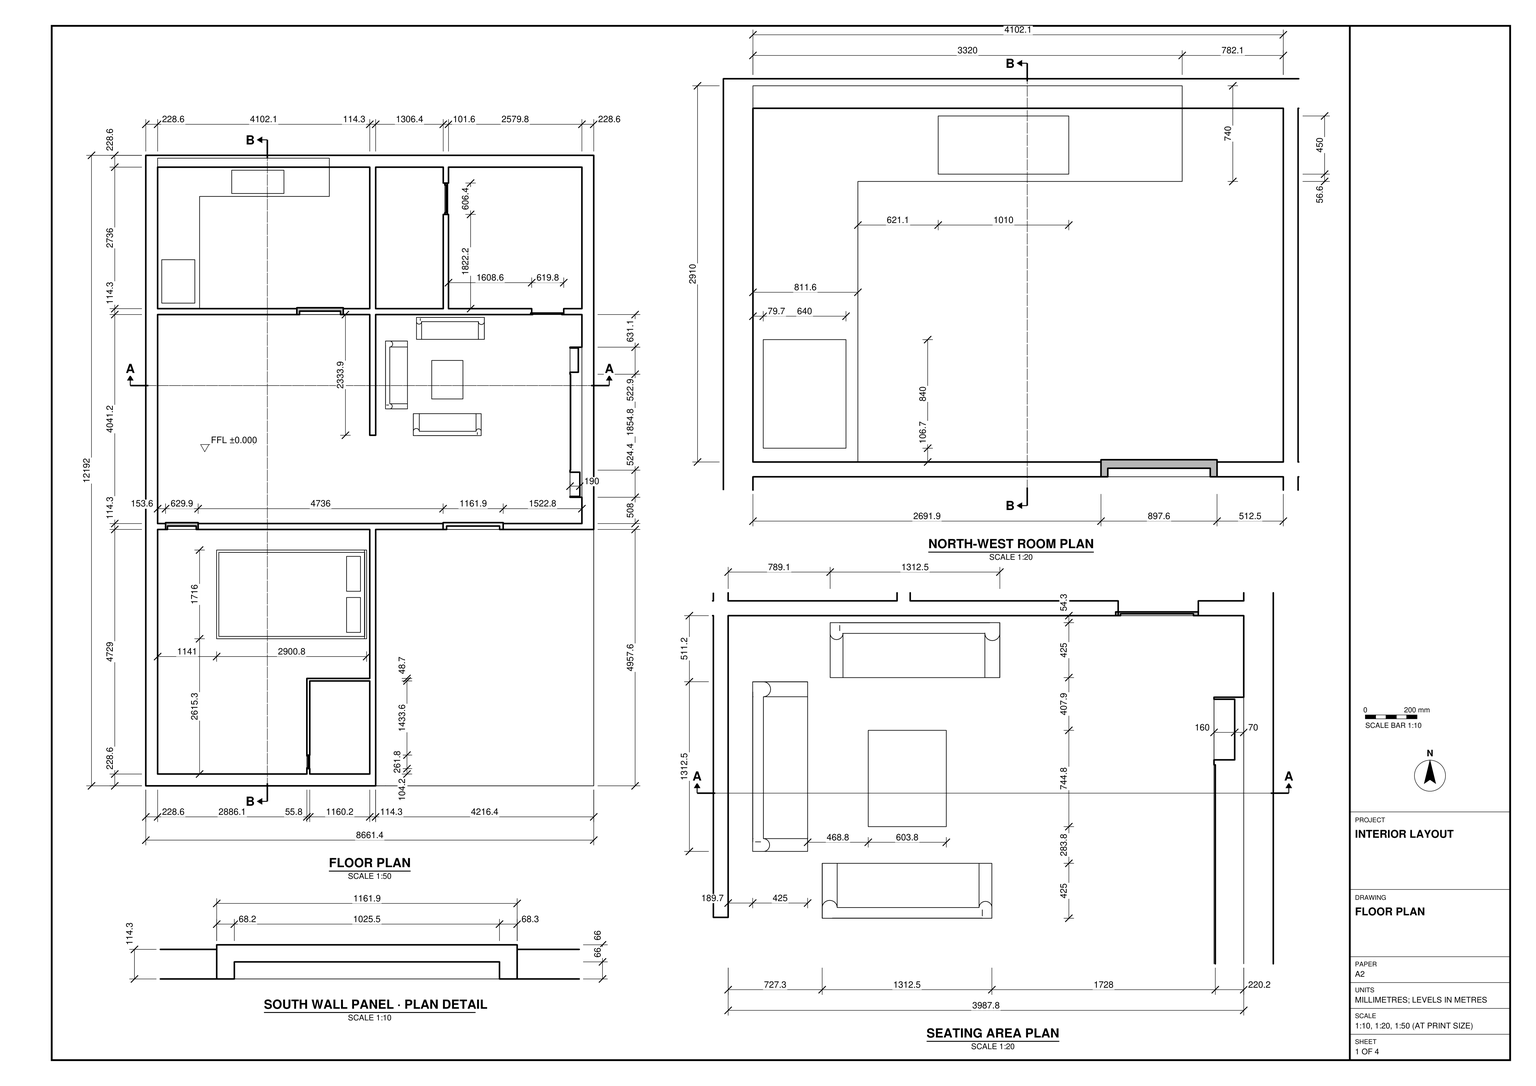
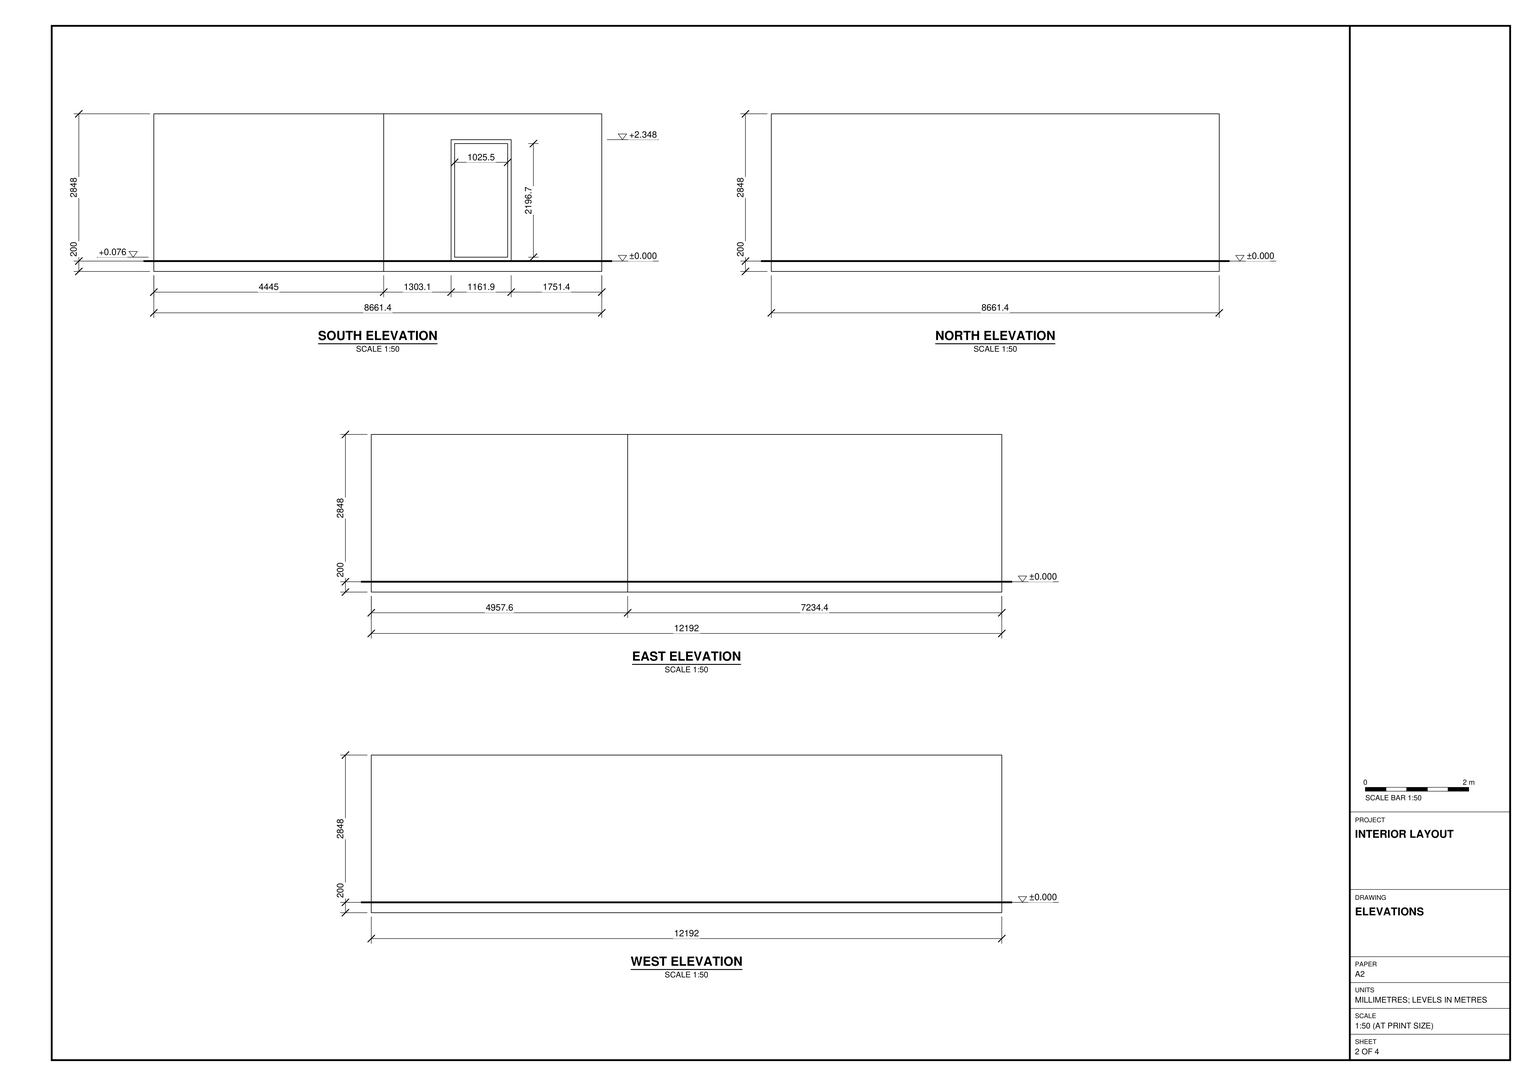
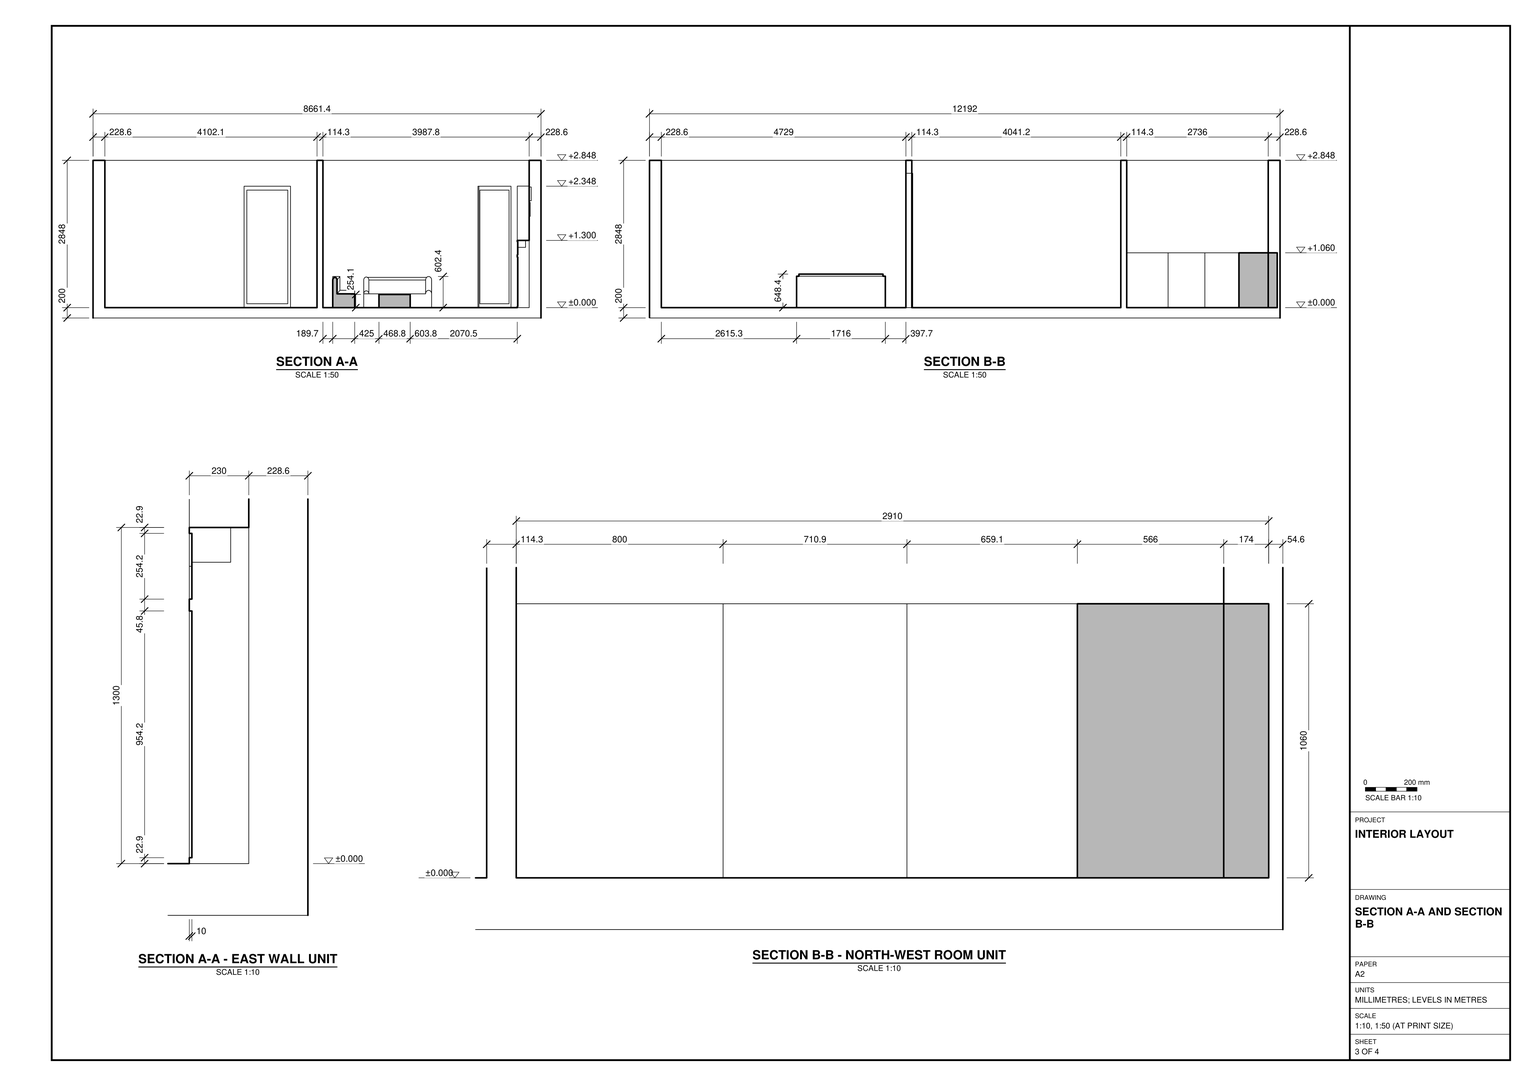
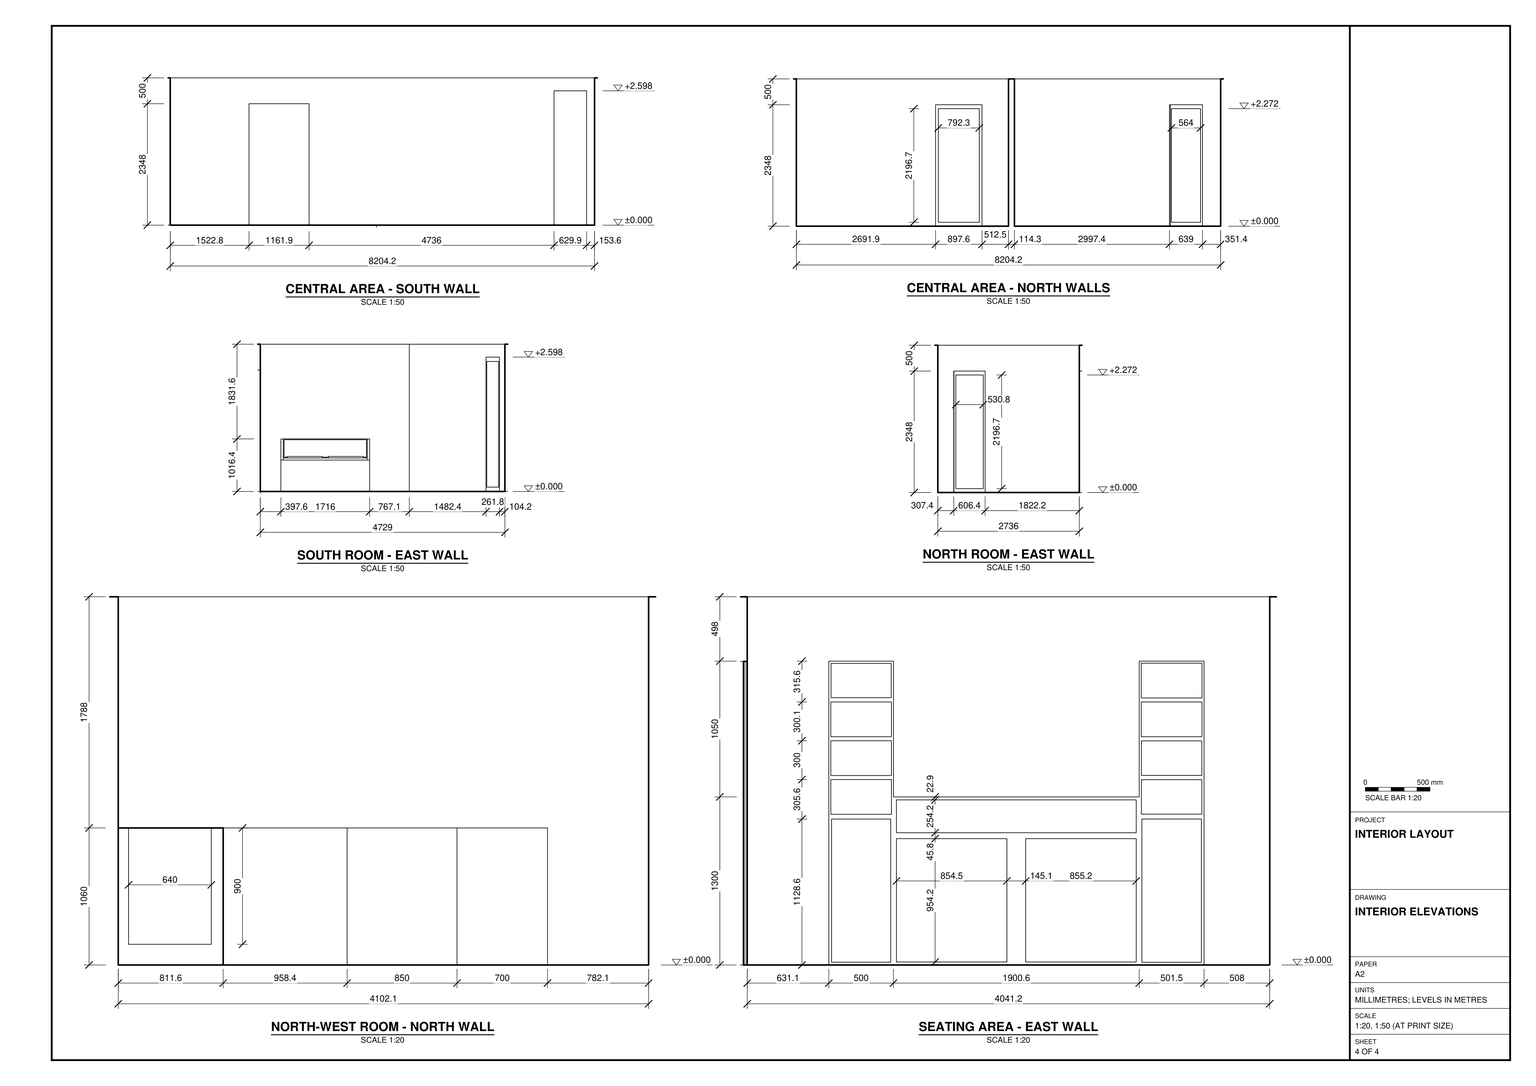
Build the interior in SketchUp from task_files/diagram_01.pdf. Work in millimetres. Set the finished floor at 0 mm and make the overall model 8661.4 mm east–west, 12192 mm north–south and 3048 mm high, including the 200 mm floor slab.

Follow the floor plan for the wall runs, thicknesses and openings. The northern row has a fitted room at the west end and two rooms to its east. In the central area, stop the dividing wall short of the south wall so the seating area remains connected to the space on its west side. Carry the bedroom south on the west side of the plan, with the bed oriented east–west and the short return partition in the bedroom corner.

Use the enlarged plans and sections to build the L-shaped unit in the north-west room, the shallow unit on the east wall and the framed panel in the south wall. Arrange the three sofas around the rectangular table as drawn. Decor and loose items shown may be any suitable library components. Keep the slab and walls separate from one another and from the fit-out. Make each furniture or joinery piece a group or component and use components for repeated parts. Save one SketchUp model as output_files/furnished_single_storey_interior_with_joinery.skp.

# SketchUp Ruby script. Lengths in millimetres.
U = 1.mm
M = Sketchup.active_model
def pt(a) = Geom::Point3d.new(a.map { |v| v * U })
def face(e, loops, mat)
  f = e.add_face(loops[0].map { |a| pt(a) })
  loops[1..].each { |l| e.add_face(l.map { |a| pt(a) }).erase! }
  f.material = f.back_material = mat if mat
  f
end
# faces: each face lists its corners as indices into pts; further lists are holes
def faces(e, pts, list, mat = nil) = list.each { |f| face(e, (f[0].is_a?(Array) ? f : [f]).map { |l| l.map { |i| pts[i] } }, mat) }
# xy, xz, yz: faces in a plane at the given z, y or x. An outline is a flat list of corners, or four numbers for a rectangle; further outlines are holes
def ring(l) = l.size == 4 ? [[l[0], l[1]], [l[2], l[1]], [l[2], l[3]], [l[0], l[3]]] : l.each_slice(2).to_a
def flat(e, list, mat, &to3) = list.each { |f| face(e, (f[0].is_a?(Array) ? f : [f]).map { |l| ring(l).map { |u, v| to3.(u, v) } }, mat) }
def xy(e, z, list, mat = nil) = flat(e, list, mat) { |x, y| [x, y, z] }
def xz(e, y, list, mat = nil) = flat(e, list, mat) { |x, z| [x, y, z] }
def yz(e, x, list, mat = nil) = flat(e, list, mat) { |y, z| [x, y, z] }
def lines(e, pts, list) = list.each { |a, b| e.add_line(pt(pts[a]), pt(pts[b])) }
# prism: a flat outline (further loops are holes) pulled along v
def prism(e, loops, v, mat = nil)
  f = face(e, loops, mat); d = Geom::Vector3d.new(v.map { |x| x * U })
  f.pushpull(f.normal.samedirection?(d) ? d.length : -d.length)
end
def box(e, o, s, mat = nil) = prism(e, [[o, [o[0] + s[0], o[1], o[2]], [o[0] + s[0], o[1] + s[1], o[2]], [o[0], o[1] + s[1], o[2]]]], [0, 0, s[2]], mat)
def at(x, y, z, deg = 0) = Geom::Transformation.translation(pt([x, y, z])) * Geom::Transformation.rotation(ORIGIN, Z_AXIS, deg.degrees)
def axes(o, x, y, z) = Geom::Transformation.new([*x, 0, *y, 0, *z, 0, *pt(o).to_a, 1])
def part(name) = M.definitions.add(name)
# library, detail: a bought-in or finely detailed component or shape, given as its bounding box
def library(name, o, s) = part(name).tap { |d| box(d.entities, o, s) }
def detail(e, o, s) = box(e.add_group.entities, o, s)
def put(e, d, t, mat = nil) = e.add_instance(d, t).tap { |i| i.material = mat if mat }
def group(e, t, mat = nil) = e.add_group.tap { |g| g.transformation = t; g.material = mat if mat }.entities
root = M.entities
M.materials.add("[Carpet Diamond Yellow]").color = [226, 217, 124]
M.materials.add("[Carpet Plush Charcoal]").color = [87, 87, 87]
M.materials.add("[Chipboard]").color = [205, 176, 119]
M.materials.add("[Color M06]").color = [86, 86, 86]
M.materials.add("[Marble Carrara Gold Floor Tile]").color = [225, 223, 217]
M.materials.add("[Plastic Red]").color = [245, 126, 1]
M.materials.add("[Resin Blue]").color = [171, 210, 241]
M.materials.add("[Resin Turquoise]").color = [117, 218, 223]
M.materials.add("[Wax 01]").color = [250, 213, 163]
M.materials.add("[Wax 02]").color = [173, 204, 163]
M.materials.add("[Wood Bamboo]").color = [177, 105, 43]
M.materials.add("[Wood Cherry Original]").color = [152, 86, 42]
c1 = part("Door panel")
xy(c1.entities,0,[[0,0,1570,60]],"[Wood Cherry Original]")
xy(c1.entities,92.1,[[92.1,0,1477.9,30]],"[Wood Cherry Original]")
xy(c1.entities,2767.9,[[92.1,0,1477.9,30]],"[Wood Cherry Original]")
xy(c1.entities,2860,[[0,0,1570,60]],"[Wood Cherry Original]")
xz(c1.entities,0,[[[0,0,1570,2860],[92.1,92.1,1477.9,2767.9]]],"[Wood Cherry Original]")
xz(c1.entities,30,[[92.1,92.1,1477.9,2767.9]],"[Wood Cherry Original]")
xz(c1.entities,60,[[0,0,1570,2860]],"[Wood Cherry Original]")
yz(c1.entities,0,[[0,0,60,2860]],"[Wood Cherry Original]")
yz(c1.entities,92.1,[[0,92.1,30,2767.9]],"[Wood Cherry Original]")
yz(c1.entities,1477.9,[[0,92.1,30,2767.9]],"[Wood Cherry Original]")
yz(c1.entities,1570,[[0,0,60,2860]],"[Wood Cherry Original]")
c2 = part("Bed with headboard")
xy(c2.entities,0,[[0,0,2860,5180]])
xy(c2.entities,1040,[[0,0,2860,0,2860,5104.1,2784.1,5104.1,2784.1,75.9,75.9,75.9,75.9,5104.1,0,5104.1]],"[Wood Cherry Original]")
xy(c2.entities,1110,[[[75.9,75.9,2784.1,5114.1],[205.2,4486.4,1330.2,4966.4],[1530.2,4486.4,2655.2,4966.4]]],"[Color M06]")
xy(c2.entities,1136.9,[[102.8,5104.1,2757.2,5114.1]])
xy(c2.entities,1160,[[205.2,4486.4,1330.2,4966.4],[1530.2,4486.4,2655.2,4966.4]],"[Color M06]")
xy(c2.entities,1713.1,[[102.8,5104.1,2757.2,5114.1]],"[Color M06]")
xy(c2.entities,1740,[[0,5104.1,75.9,5104.1,75.9,5114.1,2784.1,5114.1,2784.1,5104.1,2860,5104.1,2860,5180,0,5180]],"[Wood Cherry Original]")
xz(c2.entities,0,[[0,0,2860,1040]],"[Wood Cherry Original]")
xz(c2.entities,75.9,[[75.9,1040,2784.1,1110]],"[Color M06]")
xz(c2.entities,4486.4,[[205.2,1110,1330.2,1160],[1530.2,1110,2655.2,1160]],"[Color M06]")
xz(c2.entities,4966.4,[[205.2,1110,1330.2,1160],[1530.2,1110,2655.2,1160]])
xz(c2.entities,5104.1,[[102.8,1136.9,2757.2,1713.1]],"[Color M06]")
xz(c2.entities,5104.1,[[0,1040,75.9,1740],[2784.1,1040,2860,1740]],"[Wood Cherry Original]")
xz(c2.entities,5114.1,[[[75.9,1110,2784.1,1740],[102.8,1136.9,2757.2,1713.1]]],"[Wood Cherry Original]")
xz(c2.entities,5180,[[0,0,2860,1740]],"[Wood Cherry Original]")
yz(c2.entities,0,[[0,0,0,1040,5104.1,1040,5104.1,1740,5180,1740,5180,0]],"[Wood Cherry Original]")
yz(c2.entities,75.9,[[5104.1,1110,5114.1,1740]])
yz(c2.entities,75.9,[[75.9,1040,5104.1,1110]],"[Color M06]")
yz(c2.entities,102.8,[[5104.1,1136.9,5114.1,1713.1]],"[Color M06]")
yz(c2.entities,205.2,[[4486.4,1110,4966.4,1160]],"[Color M06]")
yz(c2.entities,1330.2,[[4486.4,1110,4966.4,1160]],"[Color M06]")
yz(c2.entities,1530.2,[[4486.4,1110,4966.4,1160]],"[Color M06]")
yz(c2.entities,2655.2,[[4486.4,1110,4966.4,1160]],"[Color M06]")
yz(c2.entities,2757.2,[[5104.1,1136.9,5114.1,1713.1]],"[Color M06]")
yz(c2.entities,2784.1,[[75.9,1040,5104.1,1110]],"[Color M06]")
yz(c2.entities,2784.1,[[5104.1,1110,5114.1,1740]],"[Wood Cherry Original]")
yz(c2.entities,2860,[[0,0,5180,0,5180,1740,5104.1,1740,5104.1,1040,0,1040]],"[Wood Cherry Original]")
c3 = part("Component\#3")
xy(c3.entities,0,[[0,0,1330,1330]])
xy(c3.entities,770,[[0,0,1330,1330]],"[Carpet Diamond Yellow]")
xz(c3.entities,0,[[0,0,1330,770]],"[Carpet Diamond Yellow]")
xz(c3.entities,1330,[[0,0,1330,770]],"[Carpet Diamond Yellow]")
yz(c3.entities,0,[[0,0,1330,770]],"[Carpet Diamond Yellow]")
yz(c3.entities,1330,[[0,0,1330,770]],"[Carpet Diamond Yellow]")
c4 = part("Upholstered sofa")
xy(c4.entities,0,[[0,0,5320,1440],[0,1440,270,1790],[270,1440,5000,1790],[5000,1440,5320,1790]])
xy(c4.entities,910,[[401.6,0,4849.7,1440]])
xy(c4.entities,1820,[[401.6,1440,4849.7,1440.5],[300,1440.5,401.6,1790]])
xz(c4.entities,0,[[0,0,5320,0,5320,910,5315.8,929.6,5310.4,970.6,5287,1027.2,5249.7,1075.7,5201.2,1112.9,5144.7,1136.3,5084,1144.3,5023.4,1136.3,4966.9,1112.9,4918.4,1075.7,4881.1,1027.2,4857.7,970.6,4849.7,910,0,910],[0,910,401.6,910,394.8,962.1,374.7,1010.7,342.7,1052.4,300.9,1084.4,252.4,1104.5,200.2,1111.4,148.1,1104.5,99.5,1084.4,57.8,1052.4,25.8,1010.7,5.7,962.1,0.8,924.9]])
xz(c4.entities,1440,[[401.6,910,4849.7,1820]])
xz(c4.entities,1790,[[0,0,0,1820,0.8,1834.9,5.7,1872.1,25.8,1920.7,57.8,1962.4,99.5,1994.4,148.1,2014.5,200.2,2021.4,252.4,2014.5,300.9,1994.4,342.7,1962.4,374.7,1920.7,394.8,1872.1,401.6,1820,5320,1820,5320,0],[4849.7,1820,4857.7,1880.6,4881.1,1937.2,4918.4,1985.7,4966.9,2022.9,5023.4,2046.3,5084,2054.3,5144.7,2046.3,5201.2,2022.9,5249.7,1985.7,5287,1937.2,5310.4,1880.6,5315.8,1839.6,5320,1820]])
yz(c4.entities,0,[[0,0,0,910,1440,910,1440,1820,1790,1820,1790,0]])
yz(c4.entities,300,[[1440.5,1820,1446.5,1865.2,1463.9,1907.2,1491.6,1943.4,1527.8,1971.1,1569.8,1988.5,1615,1994.5,1660.2,1988.5,1702.2,1971.1,1738.4,1943.4,1766.1,1907.2,1783.5,1865.2,1785.4,1851.4,1790,1820]])
yz(c4.entities,5000,[[1440.5,1820,1790,1820,1785.4,1851.4,1783.5,1865.2,1766.1,1907.2,1738.4,1943.4,1702.2,1971.1,1660.2,1988.5,1615,1994.5,1569.8,1988.5,1527.8,1971.1,1491.6,1943.4,1463.9,1907.2,1446.5,1865.2]])
yz(c4.entities,5320,[[0,0,1790,0,1790,1820,1440,1820,1440,910,0,910]])
p = [[0,0,910],[0.8,0,924.9],[0.8,1425.1,924.9],[0,1440,910],[394.8,0,962.1],[401.6,0,910],
  [401.6,1440,910],[394.8,1387.9,962.1],[4849.7,0,910],[4857.7,0,970.6],[4857.7,1379.4,970.6],[4849.7,1440,910],
  [5315.8,0,929.6],[5320,0,910],[5320,1440,910],[5315.8,1420.4,929.6],[4857.7,1379.4,1880.6],[4849.7,1440,1820],
  [401.6,1440,1820],[394.8,1387.9,1872.1],[5320,1440,1820],[5315.8,1420.4,1839.6],[0.8,1425.1,1834.9],[0,1440,1820],
  [5.7,0,962.1],[5.7,1387.9,962.1],[5.7,1387.9,1872.1],[5310.4,0,970.6],[5310.4,1379.4,970.6],[5310.4,1379.4,1880.6],
  [25.8,0,1010.7],[25.8,1339.3,1010.7],[374.7,0,1010.7],[374.7,1339.3,1010.7],[25.8,1339.3,1920.7],[374.7,1339.3,1920.7],
  [4881.1,0,1027.2],[4881.1,1322.8,1027.2],[5287,0,1027.2],[5287,1322.8,1027.2],[4881.1,1322.8,1937.2],[5287,1322.8,1937.2],
  [57.8,0,1052.4],[57.8,1297.6,1052.4],[342.7,0,1052.4],[342.7,1297.6,1052.4],[57.8,1297.6,1962.4],[342.7,1297.6,1962.4],
  [4918.4,0,1075.7],[4918.4,1274.3,1075.7],[5249.7,0,1075.7],[5249.7,1274.3,1075.7],[4918.4,1274.3,1985.7],[5249.7,1274.3,1985.7],
  [99.5,0,1084.4],[99.5,1265.6,1084.4],[300.9,0,1084.4],[300.9,1265.6,1084.4],[99.5,1265.6,1994.4],[300.9,1265.6,1994.4],
  [4966.9,0,1112.9],[4966.9,1237.1,1112.9],[5201.2,0,1112.9],[5201.2,1237.1,1112.9],[4966.9,1237.1,2022.9],[5201.2,1237.1,2022.9],
  [148.1,0,1104.5],[148.1,1245.5,1104.5],[252.4,0,1104.5],[252.4,1245.5,1104.5],[148.1,1245.5,2014.5],[252.4,1245.5,2014.5],
  [200.2,0,1111.4],[200.2,1238.6,1111.4],[200.2,1238.6,2021.4],[5023.4,0,1136.3],[5023.4,1213.7,1136.3],[5144.7,0,1136.3],
  [5144.7,1213.7,1136.3],[5023.4,1213.7,2046.3],[5144.7,1213.7,2046.3],[5084,0,1144.3],[5084,1205.7,1144.3],[5084,1205.7,2054.3],
  [4857.7,1440.5,1880.6],[4857.7,1790,1880.6],[4849.7,1790,1820],[4849.7,1440.5,1820],[401.6,1440.5,1820],[401.6,1790,1820],
  [394.8,1790,1872.1],[394.8,1440.5,1872.1],[5320,1440.5,1820],[5320,1790,1820],[5315.8,1790,1839.6],[5315.8,1440.5,1839.6],
  [0.8,1440.5,1834.9],[0.8,1790,1834.9],[0,1790,1820],[0,1440.5,1820],[5000,1446.5,1865.2],[300,1446.5,1865.2],
  [300,1440.5,1820],[5000,1440.5,1820],[300,1790,1820],[300,1785.4,1851.4],[5000,1785.4,1851.4],[5000,1790,1820],
  [5.7,1440.5,1872.1],[5.7,1790,1872.1],[5310.4,1790,1880.6],[5310.4,1440.5,1880.6],[300,1783.5,1865.2],[5000,1783.5,1865.2],
  [5000,1463.9,1907.2],[300,1463.9,1907.2],[300,1766.1,1907.2],[5000,1766.1,1907.2],[25.8,1440.5,1920.7],[25.8,1790,1920.7],
  [374.7,1790,1920.7],[374.7,1440.5,1920.7],[4881.1,1440.5,1937.2],[4881.1,1790,1937.2],[5287,1790,1937.2],[5287,1440.5,1937.2],
  [5000,1491.6,1943.4],[300,1491.6,1943.4],[300,1738.4,1943.4],[5000,1738.4,1943.4],[57.8,1440.5,1962.4],[57.8,1790,1962.4],
  [342.7,1790,1962.4],[342.7,1440.5,1962.4],[4918.4,1440.5,1985.7],[4918.4,1790,1985.7],[5249.7,1790,1985.7],[5249.7,1440.5,1985.7],
  [5000,1527.8,1971.1],[300,1527.8,1971.1],[300,1702.2,1971.1],[5000,1702.2,1971.1],[99.5,1440.5,1994.4],[99.5,1790,1994.4],
  [300.9,1790,1994.4],[300.9,1440.5,1994.4],[5000,1569.8,1988.5],[300,1569.8,1988.5],[300,1660.2,1988.5],[5000,1660.2,1988.5],
  [4966.9,1440.5,2022.9],[4966.9,1790,2022.9],[5201.2,1790,2022.9],[5201.2,1440.5,2022.9],[5000,1615,1994.5],[300,1615,1994.5],
  [148.1,1440.5,2014.5],[148.1,1790,2014.5],[252.4,1790,2014.5],[252.4,1440.5,2014.5],[200.2,1440.5,2021.4],[200.2,1790,2021.4],
  [5023.4,1440.5,2046.3],[5023.4,1790,2046.3],[5144.7,1790,2046.3],[5144.7,1440.5,2046.3],[5084,1440.5,2054.3],[5084,1790,2054.3]]
faces(c4.entities,p,[[0,1,2,3],[4,5,6,7],[8,9,10,11],[12,13,14,15],[11,10,16,17],[7,6,18,19],[15,14,20,21],[3,2,22,23],
  [1,24,25,2],[2,25,26,22],[27,12,15,28],[28,15,21,29],[24,30,31,25],[32,4,7,33],[25,31,34,26],[33,7,19,35],
  [9,36,37,10],[38,27,28,39],[10,37,40,16],[39,28,29,41],[30,42,43,31],[44,32,33,45],[31,43,46,34],[45,33,35,47],
  [36,48,49,37],[50,38,39,51],[37,49,52,40],[51,39,41,53],[42,54,55,43],[56,44,45,57],[43,55,58,46],[57,45,47,59],
  [48,60,61,49],[62,50,51,63],[49,61,64,52],[63,51,53,65],[54,66,67,55],[68,56,57,69],[55,67,70,58],[69,57,59,71],
  [66,72,73,67],[72,68,69,73],[67,73,74,70],[73,69,71,74],[60,75,76,61],[77,62,63,78],[61,76,79,64],[78,63,65,80],
  [75,81,82,76],[81,77,78,82],[76,82,83,79],[82,78,80,83],[17,16,84,85,86,87],[19,18,88,89,90,91],[21,20,92,93,94,95],[96,97,98,99,23,22],
  [100,101,102,88,87,103],[89,104,105,106,107,86],[108,109,97,96,22,26],[29,21,95,94,110,111],[106,105,112,113],[114,115,101,100],[113,112,116,117],[118,119,109,108,26,34],
  [35,19,91,90,120,121],[122,123,85,84,16,40],[41,29,111,110,124,125],[126,127,115,114],[117,116,128,129],[130,131,119,118,34,46],[47,35,121,120,132,133],[134,135,123,122,40,52],
  [53,41,125,124,136,137],[138,139,127,126],[129,128,140,141],[46,58,142,143,131,130],[59,47,133,132,144,145],[146,147,139,138],[141,140,148,149],[150,151,135,134,52,64],
  [65,53,137,136,152,153],[154,155,147,146],[149,148,155,154],[58,70,156,157,143,142],[71,59,145,144,158,159],[70,74,160,161,157,156],[74,71,159,158,161,160],[162,163,151,150,64,79],
  [153,152,164,165,80,65],[166,167,163,162,79,83],[83,80,165,164,167,166]])
c5 = library("JOSHNA.dwg",[0,0,0],[8661.4,12192,0.1])
c6 = part("L-shaped counter")
prism(c6.entities,[[[811.6,2170,0],[811.6,0,0],[0,0,0],[0,2910,0],[3320,2910,0],[3320,2170,0]]],[0,0,1060])
c7 = part("Single-storey interior")
box(c7.entities,[946.7,10150,382.4],[640,840,900])
xy(c7.entities,222.4,[[5083.4,815.9,9299.8,815.9,9299.8,5773.5,7548.5,5773.5,7548.5,5887.8,9071.2,5887.8,9071.2,6395.8,8841.2,6395.8,8841.2,9297.9,9071.2,9297.9,9071.2,9929,8719.8,9929,8719.8,10043.3,9071.2,10043.3,9071.2,12779.3,6491.4,12779.3,6491.4,12471.9,6389.8,12471.9,6389.8,12779.3,5083.4,12779.3,5083.4,10043.3,6389.8,10043.3,6389.8,11865.5,6491.4,11865.5,6491.4,10043.3,8100,10043.3,8100,9929,5083.4,9929,5083.4,7595.1,4969.1,7595.1,4969.1,9929,4456.6,9929,4456.6,10043.3,4969.1,10043.3,4969.1,12779.3,867,12779.3,867,10043.3,3558.9,10043.3,3558.9,9929,867,9929,867,5887.8,1020.6,5887.8,1020.6,5773.5,867,5773.5,867,1044.5,3753.1,1044.5,3753.1,1148.7,3808.9,1148.7,3808.9,1044.5,4969.1,1044.5,4969.1,2844.1,3808.9,2844.1,3808.9,1410.5,3753.1,1410.5,3753.1,2892.9,4969.1,2892.9,4969.1,5773.5,1650.5,5773.5,1650.5,5887.8,6386.5,5887.8,6386.5,5773.5,5083.4,5773.5]],"[Marble Carrara Gold Floor Tile]")
xy(c7.entities,245.3,[[8841.2,6920.2,8851.2,7775.4],[8841.2,7920.5,8851.2,8775]],"[Wood Bamboo]")
xy(c7.entities,1199.4,[[8841.2,6920.2,8851.2,7775.4],[8841.2,7920.5,8851.2,8775]])
xy(c7.entities,1245.3,[[8841.2,6920.2,8851.2,8775]],"[Wood Bamboo]")
xy(c7.entities,1282.4,[[2299.8,12269.9,3309.8,12719.9]])
xy(c7.entities,1387.9,[[8841.2,8813.6,9001.2,9282.3]],"[Wood Bamboo]")
xy(c7.entities,1389,[[8841.2,6412.6,9031.2,6880.5]],"[Wood Bamboo]")
xy(c7.entities,1499.4,[[8841.2,6920.2,8851.2,8775]])
xy(c7.entities,1522.4,[[8841.2,6897.3,9071.2,8797.9]],"[Wood Bamboo]")
xy(c7.entities,1655.4,[[8841.2,6412.6,9031.2,6880.5]])
xy(c7.entities,1656.6,[[8841.2,8813.6,9001.2,9282.3]])
xy(c7.entities,1687.9,[[8841.2,8813.6,9061.2,9282.3]],"[Wood Bamboo]")
xy(c7.entities,1689,[[8841.2,6412.6,9021.2,6880.5]],"[Wood Bamboo]")
xy(c7.entities,1955.4,[[8841.2,6412.6,9021.2,6880.5]])
xy(c7.entities,1956.6,[[8841.2,8813.6,9061.2,9282.3]])
xy(c7.entities,1987.9,[[8841.2,6411.4,9011.2,6881.7],[8841.2,8813.6,9091.2,9282.3]],"[Wood Bamboo]")
xy(c7.entities,2256.7,[[8841.2,6411.4,9011.2,6881.7],[8841.2,8813.6,9091.2,9282.3]])
xy(c7.entities,2288,[[8841.2,6411.4,8981.2,6881.7]],"[Wood Bamboo]")
xy(c7.entities,2289.8,[[8841.2,8815.4,9111.2,9280.5]],"[Wood Bamboo]")
xy(c7.entities,2554.9,[[8841.2,8815.4,9111.2,9280.5]])
xy(c7.entities,2556.7,[[8841.2,6411.4,8981.2,6881.7]])
xy(c7.entities,2570.4,[[6386.5,5773.5,7548.5,5887.8],[3558.9,9929,4456.6,10043.3],[8100,9929,8719.8,10043.3],[6389.8,11865.5,6491.4,12471.9]])
xy(c7.entities,2572.4,[[8841.2,6395.8,9071.2,6897.3],[8841.2,8797.9,9071.2,9297.9]],"[Wood Bamboo]")
xy(c7.entities,2820.4,[[3753.1,1148.7,3808.9,1410.5],[1020.6,5773.5,1650.5,5887.8]])
xy(c7.entities,3070.4,[[[638.4,815.9,5083.4,815.9,5083.4,5773.5,9299.8,5773.5,9299.8,13007.9,638.4,13007.9],[867,5887.8,867,9929,4969.1,9929,4969.1,7595.1,5083.4,7595.1,5083.4,9929,9071.2,9929,9071.2,5887.8],[867,1044.5,867,5773.5,4969.1,5773.5,4969.1,2892.9,3753.1,2892.9,3753.1,1044.5],[867,10043.3,4969.1,12779.3],[6491.4,10043.3,9071.2,12779.3],[5083.4,10043.3,6389.8,12779.3],[3808.9,1044.5,4969.1,2844.1]]])
xz(c7.entities,815.9,[[5083.4,22.4,9299.8,222.4]])
xz(c7.entities,815.9,[[638.4,22.4,5083.4,3070.4]],"[Wax 01]")
xz(c7.entities,1044.5,[[867,222.4,3753.1,3070.4]])
xz(c7.entities,1044.5,[[3808.9,222.4,4969.1,3070.4]],"[Plastic Red]")
xz(c7.entities,1148.7,[[3753.1,222.4,3808.9,2820.4]])
xz(c7.entities,1410.5,[[3753.1,222.4,3808.9,2820.4]])
xz(c7.entities,2844.1,[[3808.9,222.4,4969.1,3070.4]],"[Plastic Red]")
xz(c7.entities,2892.9,[[3753.1,222.4,4969.1,3070.4]],"[Resin Blue]")
xz(c7.entities,5773.5,[[867,222.4,1020.6,222.4,1020.6,2820.4,1650.5,2820.4,1650.5,222.4,4969.1,222.4,4969.1,3070.4,867,3070.4]],"[Resin Blue]")
xz(c7.entities,5773.5,[[5083.4,222.4,6386.5,222.4,6386.5,2570.4,7548.5,2570.4,7548.5,222.4,9299.8,222.4,9299.8,3070.4,5083.4,3070.4]],"[Wax 01]")
xz(c7.entities,5887.8,[[867,222.4,867,3070.4,9071.2,3070.4,9071.2,222.4,7548.5,222.4,7548.5,2570.4,6386.5,2570.4,6386.5,222.4,1650.5,222.4,1650.5,2820.4,1020.6,2820.4,1020.6,222.4]],"[Wax 02]")
xz(c7.entities,6395.8,[[8841.2,222.4,9071.2,2572.4]],"[Wood Bamboo]")
xz(c7.entities,6411.4,[[8841.2,1987.9,9011.2,2256.7],[8841.2,2288,8981.2,2556.7]],"[Wood Bamboo]")
xz(c7.entities,6412.6,[[8841.2,1389,9031.2,1655.4],[8841.2,1689,9021.2,1955.4]],"[Wood Bamboo]")
xz(c7.entities,6880.5,[[8841.2,1389,9031.2,1522.4],[8841.2,1522.4,9031.2,1655.4],[8841.2,1689,9021.2,1955.4]],"[Wood Bamboo]")
xz(c7.entities,6881.7,[[8841.2,1987.9,9011.2,2256.7],[8841.2,2288,8981.2,2556.7]],"[Wood Bamboo]")
xz(c7.entities,6897.3,[[8841.2,1522.4,9071.2,2572.4]],"[Wood Bamboo]")
xz(c7.entities,6920.2,[[8841.2,245.3,8851.2,1199.4],[8841.2,1245.3,8851.2,1372.2],[8841.2,1372.2,8851.2,1499.4]],"[Wood Bamboo]")
xz(c7.entities,7595.1,[[4969.1,222.4,5083.4,3070.4]])
xz(c7.entities,7775.4,[[8841.2,245.3,8851.2,1199.4]],"[Wood Bamboo]")
xz(c7.entities,7920.5,[[8841.2,245.3,8851.2,1199.4]],"[Wood Bamboo]")
xz(c7.entities,8775,[[8841.2,1245.3,8851.2,1372.2],[8841.2,1372.2,8851.2,1499.4]])
xz(c7.entities,8775,[[8841.2,245.3,8851.2,1199.4]],"[Wood Bamboo]")
xz(c7.entities,8797.9,[[8841.2,1522.4,9071.2,2572.4]],"[Wood Bamboo]")
xz(c7.entities,8813.6,[[8841.2,1387.9,9001.2,1522.4],[8841.2,1522.4,9001.2,1656.6],[8841.2,1687.9,9061.2,1956.6],[8841.2,1987.9,9091.2,2256.7]],"[Wood Bamboo]")
xz(c7.entities,8815.4,[[8841.2,2289.8,9111.2,2554.9]],"[Wood Bamboo]")
xz(c7.entities,9280.5,[[8841.2,2289.8,9111.2,2554.9]],"[Wood Bamboo]")
xz(c7.entities,9282.3,[[8841.2,1387.9,9001.2,1656.6],[8841.2,1687.9,9061.2,1956.6],[8841.2,1987.9,9091.2,2256.7]],"[Wood Bamboo]")
xz(c7.entities,9297.9,[[8841.2,222.4,9071.2,2572.4]],"[Wood Bamboo]")
xz(c7.entities,9929,[[867,222.4,3558.9,222.4,3558.9,2570.4,4456.6,2570.4,4456.6,222.4,4969.1,222.4,4969.1,3070.4,867,3070.4],[5083.4,222.4,8100,222.4,8100,2570.4,8719.8,2570.4,8719.8,222.4,9071.2,222.4,9071.2,3070.4,5083.4,3070.4]],"[Wax 02]")
xz(c7.entities,10043.3,[[6491.4,222.4,6491.4,3070.4,9071.2,3070.4,9071.2,222.4,8719.8,222.4,8719.8,2570.4,8100,2570.4,8100,222.4]],"[Chipboard]")
xz(c7.entities,10043.3,[[5083.4,222.4,6389.8,3070.4]],"[Plastic Red]")
xz(c7.entities,10043.3,[[867,222.4,867,3070.4,4969.1,3070.4,4969.1,222.4,4456.6,222.4,4456.6,2570.4,3558.9,2570.4,3558.9,222.4]],"[Resin Turquoise]")
xz(c7.entities,11865.5,[[6389.8,222.4,6491.4,2570.4]])
xz(c7.entities,12213.3,[[1678.6,222.4,2637,1282.4],[2637,222.4,3487,1282.4],[3487,222.4,4187,1282.4]])
xz(c7.entities,12471.9,[[6389.8,222.4,6491.4,2570.4]])
xz(c7.entities,12779.3,[[6491.4,222.4,9071.2,3070.4]],"[Chipboard]")
xz(c7.entities,12779.3,[[5083.4,222.4,6389.8,3070.4]],"[Plastic Red]")
xz(c7.entities,12779.3,[[867,222.4,4969.1,3070.4]],"[Resin Turquoise]")
xz(c7.entities,13007.9,[[638.4,22.4,9299.8,3070.4]],"[Wax 01]")
yz(c7.entities,638.4,[[815.9,22.4,13007.9,3070.4]],"[Wax 01]")
yz(c7.entities,867,[[1044.5,222.4,5773.5,3070.4]],"[Resin Blue]")
yz(c7.entities,867,[[10043.3,222.4,12779.3,3070.4]],"[Resin Turquoise]")
yz(c7.entities,867,[[5887.8,222.4,9929,3070.4]],"[Wax 02]")
yz(c7.entities,1020.6,[[5773.5,222.4,5887.8,2820.4]])
yz(c7.entities,1650.5,[[5773.5,222.4,5887.8,2820.4]])
yz(c7.entities,1678.6,[[10043.3,222.4,10843.3,1282.4],[10843.3,222.4,11554.2,1282.4],[11554.2,222.4,12213.3,1282.4]])
yz(c7.entities,3558.9,[[9929,222.4,10043.3,2570.4]])
yz(c7.entities,3753.1,[[1044.5,222.4,1044.5,3070.4,2892.9,3070.4,2892.9,222.4,1410.5,222.4,1410.5,2820.4,1148.7,2820.4,1148.7,222.4]],"[Resin Blue]")
yz(c7.entities,3808.9,[[1044.5,222.4,1148.7,222.4,1148.7,2820.4,1410.5,2820.4,1410.5,222.4,2844.1,222.4,2844.1,3070.4,1044.5,3070.4]],"[Plastic Red]")
yz(c7.entities,4456.6,[[9929,222.4,10043.3,2570.4]])
yz(c7.entities,4969.1,[[1044.5,222.4,2844.1,3070.4]],"[Plastic Red]")
yz(c7.entities,4969.1,[[2892.9,222.4,5773.5,3070.4]],"[Resin Blue]")
yz(c7.entities,4969.1,[[10043.3,222.4,12779.3,3070.4]],"[Resin Turquoise]")
yz(c7.entities,4969.1,[[7595.1,222.4,9929,3070.4]],"[Wax 02]")
yz(c7.entities,5083.4,[[10043.3,222.4,12779.3,3070.4]],"[Plastic Red]")
yz(c7.entities,5083.4,[[815.9,222.4,5773.5,3070.4]],"[Wax 01]")
yz(c7.entities,5083.4,[[7595.1,222.4,9929,3070.4]],"[Wax 02]")
yz(c7.entities,6386.5,[[5773.5,222.4,5887.8,2570.4]])
yz(c7.entities,6389.8,[[10043.3,222.4,10043.3,3070.4,12779.3,3070.4,12779.3,222.4,12471.9,222.4,12471.9,2570.4,11865.5,2570.4,11865.5,222.4]],"[Plastic Red]")
yz(c7.entities,6491.4,[[10043.3,222.4,11865.5,222.4,11865.5,2570.4,12471.9,2570.4,12471.9,222.4,12779.3,222.4,12779.3,3070.4,10043.3,3070.4]],"[Chipboard]")
yz(c7.entities,7548.5,[[5773.5,222.4,5887.8,2570.4]])
yz(c7.entities,8100,[[9929,222.4,10043.3,2570.4]])
yz(c7.entities,8719.8,[[9929,222.4,10043.3,2570.4]])
yz(c7.entities,8841.2,[[[6395.8,222.4,6395.8,2572.4,6897.3,2572.4,6897.3,1522.4,8797.9,1522.4,8797.9,2572.4,9297.9,2572.4,9297.9,222.4],[6920.2,245.3,7775.4,1199.4],[7920.5,245.3,8775,1199.4],[6416.5,243.1,6876.6,1351.5],[8819.2,243.6,9276.6,1350.9],[6920.2,1245.3,8775,1499.4],[6411.4,1987.9,6881.7,2256.7],[6411.4,2288,6881.7,2556.7],[8813.6,1987.9,9282.3,2256.7],[8813.6,1687.9,9282.3,1956.6],[8813.6,1387.9,9282.3,1656.6],[6412.6,1389,6880.5,1655.4],[6412.6,1689,6880.5,1955.4],[8815.4,2289.8,9280.5,2554.9]],[6416.5,243.1,6876.6,1351.5],[8819.2,243.6,9276.6,1350.9]],"[Wood Bamboo]")
yz(c7.entities,8851.2,[[6920.2,245.3,7775.4,1199.4],[7920.5,245.3,8775,1199.4],[6920.2,1245.3,8775,1499.4]],"[Wood Bamboo]")
yz(c7.entities,8981.2,[[6411.4,2288,6881.7,2556.7]])
yz(c7.entities,9001.2,[[8813.6,1387.9,9282.3,1656.6]])
yz(c7.entities,9011.2,[[6411.4,1987.9,6881.7,2256.7]])
yz(c7.entities,9021.2,[[6412.6,1689,6880.5,1955.4]])
yz(c7.entities,9031.2,[[6412.6,1389,6880.5,1655.4]])
yz(c7.entities,9061.2,[[8813.6,1687.9,9282.3,1956.6]])
yz(c7.entities,9071.2,[[10043.3,222.4,12779.3,3070.4]],"[Chipboard]")
yz(c7.entities,9071.2,[[5887.8,222.4,5887.8,3070.4,9929,3070.4,9929,222.4,9297.9,222.4,9297.9,2572.4,8797.9,2572.4,8797.9,1522.4,6897.3,1522.4,6897.3,2572.4,6395.8,2572.4,6395.8,222.4]],"[Wax 02]")
yz(c7.entities,9091.2,[[8813.6,1987.9,9282.3,2256.7]])
yz(c7.entities,9111.2,[[8815.4,2289.8,9280.5,2554.9]])
yz(c7.entities,9299.8,[[815.9,22.4,5773.5,222.4]])
yz(c7.entities,9299.8,[[5773.5,22.4,13007.9,3070.4]],"[Wax 01]")
put(c7.entities,c1,axes([3558.9,9929,222.4],[0.57174,0,0],[0,2.2,0],[0,0,0.82098]))
put(c7.entities,c1,axes([1020.6,5773.5,222.4],[0.4012,0,0],[0,2.2,0],[0,0,0.90839]))
put(c7.entities,c2,axes([2008,5375.9,222.4],[0,-0.6,0],[0.56,0,0],[0,0,0.58414]))
put(c7.entities,c3,axes([6167,8297,222.4],[0.45396,0,0],[0,0.56,0],[0,0,0.33]))
put(c7.entities,c4,axes([5698.1,8105.2,222.4],[0,0.24671,0],[-0.23742,0,0],[0,0,0.29325]),"[Carpet Plush Charcoal]")
put(c7.entities,c1,axes([6421.2,12466.9,222.4],[0,-0.38307,0],[0.81862,0,0],[0,0,0.82098]))
put(c7.entities,c1,axes([3753.1,1410.5,222.4],[0,-0.16677,0],[0.814,0,0],[0,0,0.90839]))
put(c7.entities,c4,axes([5872.5,9449.6,222.4],[0.24671,0,0],[0,0.23742,0],[0,0,0.29325]),"[Carpet Plush Charcoal]")
put(c7.entities,c4,axes([7123.2,8013.1,222.4],[-0.24671,0,0],[0,-0.23742,0],[0,0,0.29325]),"[Carpet Plush Charcoal]")
put(c7.entities,c5,at(638.4,815.9,22.4))
put(c7.entities,c1,axes([8080.8,9929,222.4],[0.407,0,0],[0,0.484,0],[0,0,0.82098]))
put(c7.entities,c1,axes([6386.5,5773.5,222.4],[0.74,0,0],[0,2.2,0],[0,0,0.82098]))
put(c7.entities,c6,at(867,10043.3,222.4))
put(root,c7,at(-638.4,-815.9,-22.4))
